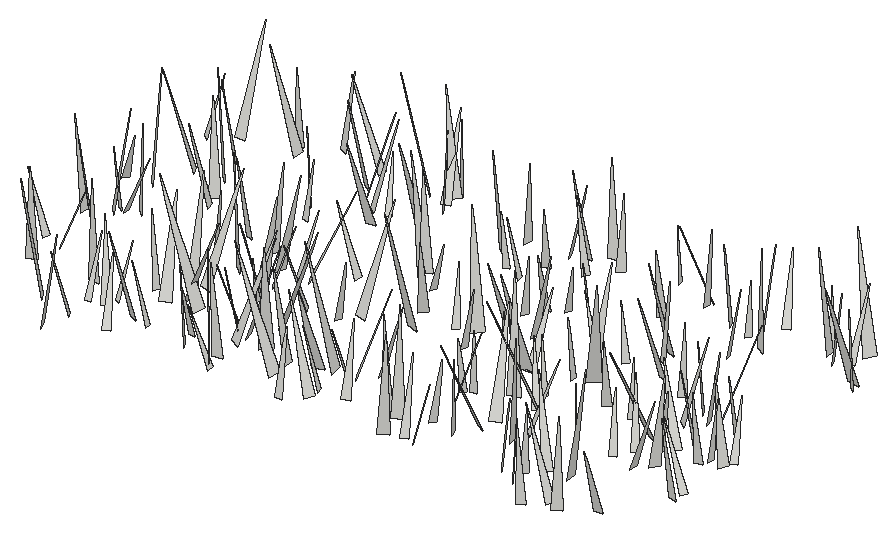
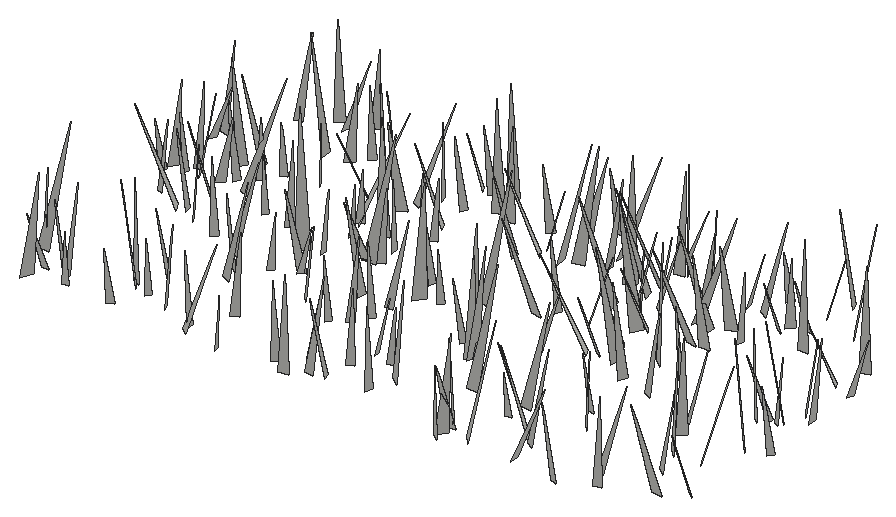
# SketchUp Ruby script. Lengths in inches.
U = 1.inch
M = Sketchup.active_model
def pt(a) = Geom::Point3d.new(a.map { |v| v * U })
def face(e, loops, mat)
  f = e.add_face(loops[0].map { |a| pt(a) })
  loops[1..].each { |l| e.add_face(l.map { |a| pt(a) }).erase! }
  f.material = f.back_material = mat if mat
  f
end
# faces: each face lists its corners as indices into pts; further lists are holes
def faces(e, pts, list, mat = nil) = list.each { |f| face(e, (f[0].is_a?(Array) ? f : [f]).map { |l| l.map { |i| pts[i] } }, mat) }
# xy, xz, yz: faces in a plane at the given z, y or x. An outline is a flat list of corners, or four numbers for a rectangle; further outlines are holes
def ring(l) = l.size == 4 ? [[l[0], l[1]], [l[2], l[1]], [l[2], l[3]], [l[0], l[3]]] : l.each_slice(2).to_a
def flat(e, list, mat, &to3) = list.each { |f| face(e, (f[0].is_a?(Array) ? f : [f]).map { |l| ring(l).map { |u, v| to3.(u, v) } }, mat) }
def xy(e, z, list, mat = nil) = flat(e, list, mat) { |x, y| [x, y, z] }
def xz(e, y, list, mat = nil) = flat(e, list, mat) { |x, z| [x, y, z] }
def yz(e, x, list, mat = nil) = flat(e, list, mat) { |y, z| [x, y, z] }
def lines(e, pts, list) = list.each { |a, b| e.add_line(pt(pts[a]), pt(pts[b])) }
# prism: a flat outline (further loops are holes) pulled along v
def prism(e, loops, v, mat = nil)
  f = face(e, loops, mat); d = Geom::Vector3d.new(v.map { |x| x * U })
  f.pushpull(f.normal.samedirection?(d) ? d.length : -d.length)
end
def box(e, o, s, mat = nil) = prism(e, [[o, [o[0] + s[0], o[1], o[2]], [o[0] + s[0], o[1] + s[1], o[2]], [o[0], o[1] + s[1], o[2]]]], [0, 0, s[2]], mat)
def at(x, y, z, deg = 0) = Geom::Transformation.translation(pt([x, y, z])) * Geom::Transformation.rotation(ORIGIN, Z_AXIS, deg.degrees)
def axes(o, x, y, z) = Geom::Transformation.new([*x, 0, *y, 0, *z, 0, *pt(o).to_a, 1])
def part(name) = M.definitions.add(name)
# library, detail: a bought-in or finely detailed component or shape, given as its bounding box
def library(name, o, s) = part(name).tap { |d| box(d.entities, o, s) }
def detail(e, o, s) = box(e.add_group.entities, o, s)
def put(e, d, t, mat = nil) = e.add_instance(d, t).tap { |i| i.material = mat if mat }
def group(e, t, mat = nil) = e.add_group.tap { |g| g.transformation = t; g.material = mat if mat }.entities
root = M.entities
c1 = part("fur_instance\#9")
p = [[0.8125,0,1.79],[0.67,-0.02,1.48],[0,-0.11,0],[0,0.11,0]]
faces(c1.entities,p,[[0,1,2,3]])
put(root,c1,axes([469.8,410.12,-21.66],[5.42096,2.25752,1.64956],[2.38588,-5.61122,-0.16143],[-1.45775,-0.7887,5.87002]))
put(root,c1,axes([536.05,411.73,-21.66],[-1.45922,4.42701,2.15741],[4.90506,1.50733,0.22462],[0.43952,-2.12407,4.65589]))
put(root,c1,axes([540.0625,413.08,-21.66],[2.8988,-5.16102,2.16058],[-5.5292,-3.01461,0.21733],[-0.85564,1.9958,5.91539]))
put(root,c1,axes([470.66,413.89,-21.66],[-3.26871,-2.2439,0.63682],[-2.29753,3.28654,-0.21245],[0.40248,0.53729,3.95909]))
put(root,c1,axes([490.34,414.11,-21.66],[-3.97846,-0.22397,0.26493],[-0.21326,3.98441,0.16592],[0.27363,-0.15114,3.9813]))
put(root,c1,axes([543.85,415.63,-21.66],[0.47232,-5.02453,0.37853],[-5.03579,-0.45765,0.20889],[0.17316,0.39615,5.04235]))
put(root,c1,axes([514.4,414.54,-21.66],[4.01557,-5.25956,2.05629],[-5.53772,-4.16187,0.169],[-1.10676,1.74125,6.61508]))
put(root,c1,axes([500.37,413.59,-21.66],[0.04059,4.23783,1.33242],[4.44047,0.00019,-0.13586],[0.12965,-1.33303,4.23585]))
put(root,c1,axes([538.44,413.93,-21.66],[-5.80532,1.01557,0.17125],[1.00882,5.80466,-0.22508],[0.20737,0.19232,5.88918]))
put(root,c1,axes([465.71,415.29,-21.66],[-6.16765,-3.82155,1.90605],[-3.98751,6.35208,-0.16723],[1.52874,1.15063,7.2537]))
put(root,c1,axes([532.24,415.05,-21.66],[-2.65775,-2.55388,1.91088],[-2.80676,3.05414,0.17806],[1.51521,1.17784,3.68161]))
put(root,c1,axes([476.0625,413.6875,-21.66],[-2.52047,3.62206,0.22803],[3.61381,2.53037,-0.24846],[0.33426,-0.04477,4.40572]))
put(root,c1,axes([489.03,415.52,-21.66],[4.97701,4.02381,2.97396],[4.34378,-5.5566,0.24873],[-2.48337,-1.65505,6.3953]))
put(root,c1,axes([518.21,415.05,-21.66],[2.97809,2.23148,0.68885],[2.24903,-3.04112,0.12836],[-0.62921,-0.30835,3.71915]))
put(root,c1,axes([489.35,416.62,-21.66],[1.40139,-5.88916,2.09043],[-6.21682,-1.53152,-0.14692],[-0.635,1.99706,6.05182]))
put(root,c1,axes([516.77,415.28,-21.66],[-2.07994,4.49979,1.08625],[4.57933,2.1742,-0.23818],[0.67657,-0.88257,4.95151]))
put(root,c1,axes([484.82,416.42,-21.66],[-3.86454,-2.68359,1.87384],[-2.96857,4.09497,-0.25773],[1.3786,1.29506,4.69786]))
put(root,c1,axes([502.83,415.91,-21.66],[-5.78073,2.46703,0.60773],[2.49572,5.79658,0.20851],[0.47643,-0.43109,6.28168]))
put(root,c1,axes([476.64,417.7,-21.66],[-2.84226,-5.05917,1.08036],[-5.16298,2.85167,-0.22901],[0.32566,1.05526,5.79838]))
put(root,c1,axes([529.49,416.57,-21.66],[3.10895,3.01642,1.49943],[3.22004,-3.26039,-0.11754],[-0.98914,-1.13301,4.33019]))
put(root,c1,axes([531.97,417.37,-21.66],[2.86459,-3.18276,1.27512],[-3.34476,-2.95943,0.1272],[-0.754,1.03614,4.28015]))
put(root,c1,axes([479.02,417.29,-21.66],[-3.86057,-0.50737,0.50019],[-0.53854,3.88252,-0.21837],[0.46646,0.28336,3.88764]))
put(root,c1,axes([496.76,417.38,-21.66],[-8.06825,0.70999,0.37952],[0.71569,8.07597,0.10667],[0.36866,-0.13964,8.09873]))
put(root,c1,axes([484.07,418.64,-21.66],[-0.05824,-3.81958,0.55077],[-3.85535,0.08183,0.15984],[0.16986,0.54776,3.81668]))
put(root,c1,axes([502.81,417.75,-21.66],[-3.79015,-1.11399,0.60809],[-1.15598,3.82064,-0.20588],[0.52388,0.37109,3.9451]))
put(root,c1,axes([513.49,418.23,-21.66],[-2.45983,6.23998,3.07468],[6.83629,2.77173,-0.15592],[1.28687,-2.79677,6.7055]))
put(root,c1,axes([506.4,417.93,-21.66],[-1.7521,4.37342,1.24469],[4.49457,1.86786,-0.23622],[0.6891,-1.06311,4.7054]))
put(root,c1,axes([511.42,418.98,-21.66],[-0.9402,5.50023,2.63792],[6.09336,0.97222,0.14463],[0.28664,-2.62629,5.57814]))
put(root,c1,axes([470.32,417.61,-21.66],[0.12612,4.07155,0.3622],[4.08216,-0.1442,0.19951],[-0.2114,-0.35539,4.06861]))
put(root,c1,axes([499.63,421.51,-21.66],[2.0561,-6.44135,0.2848],[-6.4395,-2.06652,-0.24899],[-0.32395,0.19535,6.75697]))
put(root,c1,axes([472.42,418.19,-21.66],[-4.08375,3.22336,1.0157],[3.24667,4.18417,-0.22495],[0.93853,-0.4488,5.19774]))
put(root,c1,axes([520.35,419.51,-21.66],[4.15283,1.56186,1.94961],[1.7605,-4.5132,-0.13443],[-1.7723,-0.82343,4.43479]))
put(root,c1,axes([536.68,419.74,-21.66],[7.17764,0.6661,2.04171],[0.73913,-7.45363,-0.1667],[-2.01642,-0.36113,7.20655]))
put(root,c1,axes([517.06,420,-21.66],[3.70956,-2.15387,1.10856],[-2.28011,-3.78925,0.26761],[-0.81802,0.79458,4.28116]))
put(root,c1,axes([496.37,420.23,-21.66],[-5.73495,-0.11109,1.68244],[-0.04447,5.97258,0.24275],[1.68552,-0.22038,5.73089]))
put(root,c1,axes([533.68,419.23,-21.66],[-4.18107,4.06515,1.12452],[4.17237,4.21812,0.26475],[0.61747,-0.97641,5.82552]))
put(root,c1,axes([521.83,422.34,-21.66],[-3.10911,-5.59083,0.18925],[-5.58666,3.11434,0.22319],[0.28707,0.05678,6.39328]))
put(root,c1,axes([492.43,421.375,-21.66],[4.53182,-5.76132,1.66498],[-5.89155,-4.66684,-0.11276],[-1.12014,1.237,7.32923]))
put(root,c1,axes([504.39,421.02,-21.66],[-3.02688,-2.08558,0.64094],[-2.07151,3.09116,0.27563],[0.68504,0.13224,3.66547]))
put(root,c1,axes([459.58,421.11,-21.66],[2.04038,-5.82637,1.87095],[-6.1057,-2.07021,0.21174],[-0.4092,1.83789,6.16967]))
put(root,c1,axes([472.86,419.62,-21.66],[1.48501,3.27806,0.44782],[3.28348,-1.52047,0.24164],[-0.40618,-0.30651,3.59062]))
put(root,c1,axes([468,421.49,-21.66],[0.12589,-6.48138,2.39431],[-6.90548,-0.03647,0.26437],[0.23531,2.39734,6.47721]))
put(root,c1,axes([501.4,422.42,-21.66],[-7.78363,-1.77881,1.5879],[-1.77027,7.9428,0.22014],[1.59741,0.13482,7.98126]))
put(root,c1,axes([548.46,422.96,-21.66],[-1.20745,-5.31811,1.49773],[-5.50418,1.29079,0.14593],[0.47907,1.42653,5.45151]))
put(root,c1,axes([526.46,422.29,-21.66],[-5.78196,-1.74059,3.08913],[-1.82129,6.52793,0.26926],[3.04225,0.59997,6.03227]))
put(root,c1,axes([487.04,423.0625,-21.66],[2.58883,2.26123,2.35644],[2.87323,-3.00647,-0.27159],[-1.55259,-1.79333,3.42658]))
put(root,c1,axes([488.87,420.32,-21.66],[3.08355,6.47581,0.56476],[6.50039,-3.07095,-0.27862],[0.00972,-0.62967,7.16706]))
put(root,c1,axes([489.17,422.3,-21.66],[6.39922,1.66084,0.77373],[1.68967,-6.43637,-0.15871],[-0.70856,-0.34898,6.60932]))
put(root,c1,axes([486.41,424.06,-21.66],[-2.51428,-3.3921,0.48717],[-3.39486,2.54791,0.21985],[0.4675,0.25907,4.21659]))
put(root,c1,axes([481.19,423.55,-21.66],[-8.2127,0.65784,0.53458],[0.66874,8.22786,0.14871],[0.52088,-0.19122,8.23766]))
put(root,c1,axes([504.21,422.53,-21.66],[4.71146,3.59222,0.48874],[3.58656,-4.73541,0.23065],[-0.52868,-0.11206,5.92019]))
put(root,c1,axes([478.84,424.3,-21.66],[6.32916,0.13104,0.27334],[0.13733,-6.3333,-0.14369],[-0.27023,-0.14945,6.32889]))
put(root,c1,axes([477.09,422.76,-21.66],[-2.49742,5.95651,1.04282],[6.02179,2.55284,-0.16018],[0.55273,-0.89868,6.45689]))
put(root,c1,axes([474.625,424.23,-21.66],[-4.53937,1.16522,1.40638],[1.15678,4.75002,-0.2018],[1.41333,-0.14527,4.6822]))
put(root,c1,axes([516.41,424.4,-21.66],[4.75078,2.28793,0.55209],[2.32197,-4.75936,-0.25743],[-0.38451,-0.47246,5.26671]))
put(root,c1,axes([506.1,424.72,-21.66],[4.91416,0.05831,0.74386],[0.02898,-4.96646,0.19783],[-0.74558,0.19125,4.91052]))
put(root,c1,axes([548.78,424.58,-21.66],[-4.27711,1.68369,0.0136],[1.68167,4.26988,0.26227],[-0.08344,-0.24902,4.58909]))
put(root,c1,axes([533.05,425.26,-21.66],[3.08289,1.97486,1.70839],[2.08981,-3.45082,0.21788],[-1.56569,-0.71742,3.6547]))
put(root,c1,axes([540.625,425.82,-21.66],[5.32067,-0.59583,0.38531],[-0.58759,-5.33383,-0.13414],[-0.39777,-0.09079,5.35224]))
put(root,c1,axes([487.4,425.89,-21.66],[2.96101,1.91002,1.7712],[2.18546,-3.28075,-0.11568],[-1.41742,-1.06838,3.5217]))
put(root,c1,axes([526.92,424.48,-21.66],[2.95968,3.81178,0.17357],[3.80838,-2.96454,0.16477],[-0.23661,-0.0359,4.82309]))
put(root,c1,axes([457.63,426.06,-21.66],[-4.13289,0.76106,0.51137],[0.79822,4.14817,0.27763],[0.45116,-0.36746,4.1932]))
put(root,c1,axes([460.37,425.12,-21.66],[3.48298,2.03603,0.22687],[2.02285,-3.48877,0.25421],[-0.32396,0.10555,4.02641]))
put(root,c1,axes([522.31,424.4,-21.66],[-2.78795,6.31949,0.96814],[6.36227,2.84625,-0.25738],[0.62828,-0.78026,6.90234]))
put(root,c1,axes([515.3,427.45,-21.66],[2.03457,-2.99845,1.01926],[-3.06758,-2.16697,-0.25148],[-0.78708,0.69471,3.61482]))
put(root,c1,axes([490.62,426.48,-21.66],[6.76067,1.19839,0.69108],[1.18973,-6.79585,0.14582],[-0.7059,0.02372,6.86451]))
put(root,c1,axes([542.37,427.46,-21.66],[5.43979,-3.16023,1.66658],[-3.30816,-5.60189,0.17546],[-1.34931,0.9938,6.28869]))
put(root,c1,axes([537.27,426.45,-21.66],[-1.47,3.64091,0.87512],[3.73843,1.4809,0.11844],[0.21496,-0.85654,3.92467]))
put(root,c1,axes([486.72,428.26,-21.66],[-4.48858,-3.56813,1.07524],[-3.58767,4.5928,0.2643],[1.00813,0.45789,5.72792]))
put(root,c1,axes([524.41,429.38,-21.66],[-5.605,-5.08718,0.25266],[-5.09303,5.60246,-0.18084],[0.06544,0.30374,7.56721]))
put(root,c1,axes([516.32,428,-21.66],[0.16475,-3.83195,1.51207],[-4.1166,-0.0965,0.20397],[0.15418,1.51796,3.83006]))
put(root,c1,axes([485.19,429.32,-21.66],[6.75458,-3.1446,1.55563],[-3.25939,-6.87331,0.25842],[-1.29802,0.89549,7.44621]))
put(root,c1,axes([476.94,427.67,-21.66],[-0.4945,6.57851,1.5324],[6.75453,0.47319,0.14829],[-0.03697,-1.53911,6.5954]))
put(root,c1,axes([538.65,428.65,-21.66],[-2.21571,3.96483,0.99922],[4.07213,2.24229,0.13245],[0.36886,-0.93805,4.54001]))
put(root,c1,axes([538.22,432.16,-21.66],[-2.55623,-6.61752,0.06611],[-6.61278,2.55692,0.25211],[0.25899,-0.02922,7.08959]))
put(root,c1,axes([484.28,428.47,-21.66],[3.52648,2.43175,0.31475],[2.41999,-3.54045,0.23962],[-0.3951,0.0194,4.27692]))
put(root,c1,axes([540.69,430.41,-21.66],[4.29298,-1.68508,0.76366],[-1.68331,-4.35833,-0.1541],[-0.76754,0.13347,4.60928]))
put(root,c1,axes([545.64,430.99,-21.66],[1.04102,-4.92803,1.21287],[-5.07408,-1.03535,0.14838],[-0.10125,1.21771,5.0346]))
put(root,c1,axes([524.11,429.34,-21.66],[-2.51117,3.39602,0.58609],[3.43959,2.51478,0.1658],[0.21361,-0.57041,4.22035]))
put(root,c1,axes([478.67,427.8,-21.66],[1.55056,7.17303,0.47228],[7.18686,-1.53634,-0.26142],[0.15632,-0.51668,7.33405]))
put(root,c1,axes([490.3125,431.25,-21.66],[-3.61255,-2.36918,0.54232],[-2.35627,3.65218,0.25916],[0.59592,0.07847,4.31235]))
put(root,c1,axes([520.34,430.09,-21.66],[1.64686,-6.77743,3.62945],[-7.62252,-1.92308,-0.13234],[-1.0018,3.49096,6.97339]))
put(root,c1,axes([494.48,431.53,-21.66],[4.0424,-1.6774,0.68877],[-1.67315,-4.09915,-0.16314],[-0.69903,0.11126,4.37357]))
put(root,c1,axes([544.71,431.93,-21.66],[-4.89111,-2.11302,1.38613],[-2.21595,5.03778,-0.13961],[1.21481,0.68196,5.3262]))
put(root,c1,axes([517.23,432.02,-21.66],[4.14484,0.5886,1.74948],[0.68446,-4.48393,-0.11303],[-1.71425,-0.36717,4.1849]))
put(root,c1,axes([546.34,432.375,-21.66],[4.13906,-0.88394,1.08396],[-0.87234,-4.27812,-0.15771],[-1.09332,0.06702,4.22946]))
put(root,c1,axes([548.3,432.09,-21.66],[-4.8782,2.33838,1.88669],[2.5546,5.12175,0.25721],[1.58166,-1.06025,5.40358]))
put(root,c1,axes([458.8125,432.4,-21.66],[3.31439,2.62679,2.62231],[3.03004,-3.94532,0.12232],[-2.14367,-1.5153,4.22732]))
put(root,c1,axes([523.06,432.22,-21.66],[3.01506,-0.72225,2.0256],[-1.00024,-3.559,0.21985],[-1.90373,0.72607,3.09256]))
put(root,c1,axes([541.875,431.86,-21.66],[-4.34264,3.05124,0.46122],[3.07623,4.34339,0.23041],[0.24406,-0.45414,5.3024]))
put(root,c1,axes([478.83,433.39,-21.66],[-4.49865,-5.44108,2.87885],[-5.83326,4.90701,0.15896],[1.96626,2.10876,7.05818]))
put(root,c1,axes([502.04,435.15,-21.66],[-2.39726,-7.68863,1.50052],[-7.81274,2.46126,0.12966],[0.5725,1.39306,8.05265]))
put(root,c1,axes([517.87,435.57,-21.66],[0.49777,-7.47829,0.86543],[-7.52286,-0.52678,-0.22508],[-0.28353,0.84808,7.49146]))
put(root,c1,axes([457.3,433.2,-21.66],[4.90342,0.51596,3.18153],[0.4361,-5.84514,0.27581],[-3.19346,-0.00597,4.92277]))
put(root,c1,axes([484.25,432.74,-21.66],[3.13129,2.44329,0.37399],[2.42945,-3.15346,0.26073],[-0.45532,-0.0231,3.96316]))
put(root,c1,axes([529.62,434.91,-21.66],[3.06125,-3.87557,0.82155],[-3.90702,-3.12527,-0.1848],[-0.65588,0.52812,4.93529]))
put(root,c1,axes([474.8,434.57,-21.66],[4.07501,0.67414,1.38281],[0.80205,-4.27202,-0.28088],[-1.31276,-0.5174,4.12083]))
put(root,c1,axes([548.76,433.41,-21.66],[-1.59242,3.59476,0.56652],[3.61736,1.63113,-0.18207],[0.39739,-0.44291,3.92746]))
put(root,c1,axes([533.58,434.28,-21.66],[-2.47,2.58512,1.49197],[2.74392,2.72878,-0.18549],[1.17462,-0.93843,3.57063]))
put(root,c1,axes([509.375,435.13,-21.66],[4.26328,-1.39926,0.74192],[-1.39292,-4.32659,-0.15583],[-0.75375,0.08115,4.48433]))
put(root,c1,axes([516.62,435.02,-21.66],[2.27684,-3.73592,1.683],[-3.94498,-2.51908,-0.25488],[-1.10756,1.29258,4.36763]))
put(root,c1,axes([496.08,433.37,-21.66],[1.83288,7.01444,0.75411],[7.05484,-1.82448,-0.17632],[-0.01908,-0.77421,7.24781]))
put(root,c1,axes([460.07,436.02,-21.66],[-1.89592,-3.45095,1.30694],[-3.60556,2.04518,0.16982],[0.78554,1.05823,3.9338]))
put(root,c1,axes([459.89,435.1,-21.66],[-4.21577,-3.58718,3.5566],[-4.31781,4.96325,-0.11214],[2.62178,2.40587,5.53425]))
put(root,c1,axes([482.59,436.15,-21.66],[6.6153,-1.38256,1.33275],[-1.44359,-6.733,0.18083],[-1.26639,0.45296,6.75581]))
put(root,c1,axes([525.23,438.07,-21.66],[5.72891,-5.77899,0.7373],[-5.79412,-5.75966,-0.12335],[-0.60698,0.43635,8.13646]))
put(root,c1,axes([460.98,435.99,-21.66],[4.07736,0.20577,0.16386],[0.20057,-4.0788,0.13116],[-0.17019,0.12285,4.08044]))
put(root,c1,axes([462.42,436.74,-21.66],[-3.23296,-4.09809,2.47034],[-4.47809,3.64184,0.18098],[1.68632,1.81429,5.21667]))
put(root,c1,axes([523.06,437.2,-21.66],[3.59976,0.06174,1.80471],[0.19659,-4.01441,-0.2548],[-1.79504,-0.31584,3.59126]))
put(root,c1,axes([545.87,437.55,-21.66],[-1.67476,-3.89018,1.26522],[-4.03938,1.78862,0.15259],[0.64624,1.09838,4.23261]))
put(root,c1,axes([485.2,436.09,-21.66],[2.13777,3.57515,0.4757],[3.58502,-2.16686,0.17428],[-0.39447,-0.3179,4.1619]))
put(root,c1,axes([500.69,438.7,-21.66],[3.52243,-4.25283,0.7835],[-4.27225,-3.57882,-0.21878],[-0.66956,0.46198,5.5178]))
put(root,c1,axes([518.39,435.48,-21.66],[-0.5351,4.97369,0.08314],[4.96853,0.53845,-0.2337],[0.24128,-0.05757,4.99693]))
put(root,c1,axes([486.43,436.48,-21.66],[5.74165,3.30721,0.02247],[3.30582,-5.73764,-0.2359],[0.09829,-0.21562,6.62182]))
put(root,c1,axes([538.85,436.68,-21.66],[-2.72966,-3.54913,3.67888],[-4.47058,3.67982,0.23296],[2.47878,2.72838,4.47136]))
put(root,c1,axes([505.9,437.97,-21.66],[-2.49672,2.92464,0.96124],[2.97957,2.60694,-0.1927],[0.77439,-0.6012,3.84057]))
put(root,c1,axes([540.94,438.84,-21.66],[4.61454,1.12705,1.27743],[1.23829,-4.75228,-0.2803],[-1.16993,-0.58453,4.7419]))
put(root,c1,axes([479.63,438.72,-21.66],[5.47744,-1.647,1.93505],[-1.81976,-5.75174,0.25556],[-1.77356,0.81501,5.71398]))
put(root,c1,axes([508.29,438.75,-21.66],[5.58768,-4.04107,3.86555],[-4.58295,-6.44048,-0.10822],[-3.20457,2.16447,6.89498]))
put(root,c1,axes([475.3,439.76,-21.66],[-2.10468,-4.52268,1.53831],[-4.75533,2.14388,-0.20306],[0.45584,1.48319,4.98428]))
put(root,c1,axes([539,440.18,-21.66],[-3.54566,-2.66431,1.6705],[-2.78653,3.82874,0.19209],[1.45754,0.83849,4.43096]))
put(root,c1,axes([490.47,440.07,-21.66],[-4.67838,0.58429,0.4377],[0.60816,4.68963,0.24018],[0.40387,-0.29353,4.7086]))
put(root,c1,axes([509.77,442.29,-21.66],[-0.22883,-5.12281,0.23524],[-5.12454,0.23734,0.18366],[0.19416,0.22665,5.12463]))
put(root,c1,axes([542.21,439.14,-21.66],[6.025,3.41302,0.55167],[3.40656,-6.04972,0.22351],[-0.59027,-0.07668,6.92094]))
put(root,c1,axes([456.22,441.83,-21.66],[3.1539,-2.32332,0.00557],[-2.32207,-3.15188,0.13648],[0.07647,0.11319,3.91488]))
put(root,c1,axes([534.94,441.6,-21.66],[-2.61332,3.50076,2.27341],[3.90248,3.00092,-0.13507],[1.48133,-1.72983,4.36652]))
put(root,c1,axes([513.8,442.01,-21.66],[5.74343,-0.59024,1.12729],[-0.57342,-5.85294,-0.14303],[-1.13593,-0.02976,5.77191]))
put(root,c1,axes([530.66,443.48,-21.66],[-1.81224,-5.34948,0.90018],[-5.42401,1.80193,-0.21131],[0.08596,0.92064,5.64415]))
put(root,c1,axes([467.42,442.65,-21.66],[-4.87581,-1.54153,0.97742],[-1.54685,4.96967,0.12147],[0.96896,0.17664,5.11224]))
put(root,c1,axes([498.44,443.34,-21.66],[3.31097,-1.72543,0.32906],[-1.73993,-3.31791,0.10944],[-0.24091,0.24944,3.73197]))
put(root,c1,axes([522.26,442.32,-21.66],[-3.36159,2.04077,0.19725],[2.04893,3.35754,0.1809],[0.07444,-0.25709,3.9284]))
put(root,c1,axes([459.37,442.58,-21.66],[4.78863,4.89843,2.46119],[5.13986,-5.14824,0.24599],[-1.90629,-1.57608,6.84581]))
put(root,c1,axes([522.34,441.88,-21.66],[-0.07417,5.83715,1.21265],[5.95855,0.11247,-0.17697],[0.19614,-1.2097,5.83493]))
put(root,c1,axes([525.3125,443.69,-21.66],[-2.21806,2.84038,1.31516],[3.07662,2.27502,0.2754],[0.57601,-1.21396,3.59328]))
put(root,c1,axes([509.79,445.23,-21.66],[3.72524,-2.31212,0.81738],[-2.32656,-3.80205,-0.15146],[-0.77532,0.29988,4.38182]))
put(root,c1,axes([466.73,444.4375,-21.66],[3.45962,-4.50001,2.91683],[-5.02174,-3.93643,-0.1168],[-1.88153,2.2319,5.67498]))
put(root,c1,axes([495.38,445.46,-21.66],[-7.11208,1.53537,2.26223],[1.65379,7.4363,0.15223],[2.17716,-0.6331,7.27433]))
put(root,c1,axes([495.52,445.7,-21.66],[3.10657,-5.20372,2.6425],[-5.63717,-3.45056,-0.16782],[-1.51121,2.17421,6.05816]))
put(root,c1,axes([511.11,447.47,-21.66],[1.53045,-4.60076,0.23907],[-4.60681,-1.52625,0.11946],[0.03806,0.26453,4.84716]))
put(root,c1,axes([518.17,446.57,-21.66],[-3.06281,-3.15709,1.43812],[-3.29391,3.24851,0.11628],[1.08883,0.94666,4.3971]))
put(root,c1,axes([528.46,446.27,-21.66],[-2.24155,-3.80564,2.54295],[-4.42537,2.52493,-0.12217],[1.16862,2.26183,4.41503]))
put(root,c1,axes([461.24,447.79,-21.66],[-5.49942,-3.45806,0.94275],[-3.51329,5.5426,-0.16378],[0.70973,0.64178,6.49422]))
put(root,c1,axes([477.7,446.68,-21.66],[1.06055,3.50039,1.15885],[3.68372,-1.05849,-0.17402],[-0.16095,-1.16074,3.65339]))
put(root,c1,axes([527.93,448.32,-21.66],[-2.71876,-5.31687,1.33657],[-5.469,2.73415,-0.24823],[0.3815,1.3048,5.9665]))
put(root,c1,axes([464.92,448.27,-21.66],[4.55418,4.59674,3.34406],[5.23121,-5.06575,-0.16086],[-2.22422,-2.50228,6.46875]))
put(root,c1,axes([513.14,448.69,-21.66],[3.09975,-1.98369,0.33098],[-1.98147,-3.11644,-0.1208],[-0.34401,0.07615,3.67817]))
put(root,c1,axes([483.9,450.47,-21.66],[0.0355,-6.28923,0.69696],[-6.32457,-0.05728,-0.19472],[-0.19984,0.69551,6.28631]))
put(root,c1,axes([491.09,450.92,-21.66],[-1.0754,-7.3325,1.08617],[-7.40599,1.10888,0.15329],[0.31086,1.05196,7.40935]))
put(root,c1,axes([475.96,449.7,-21.66],[3.3067,2.95122,2.18217],[3.23124,-3.73382,0.15332],[-1.74087,-1.32466,4.4295]))
put(root,c1,axes([504.39,451.2,-21.66],[-3.7389,-0.44853,0.79303],[-0.43438,3.82202,0.11371],[0.80087,-0.02096,3.764]))
put(root,c1,axes([463.32,452.23,-21.66],[-2.97615,-4.05495,1.48787],[-4.26463,3.04523,-0.23114],[0.68511,1.34083,5.02461]))
put(root,c1,axes([501.67,452.18,-21.66],[0.6335,-3.36408,1.34348],[-3.58683,-0.77327,-0.24494],[-0.50657,1.2682,3.41444]))
put(root,c1,axes([533.28,451.81,-21.66],[4.00682,1.30969,1.18737],[1.29487,-4.17692,0.23764],[-1.20352,-0.13365,4.20874]))
put(root,c1,axes([547.74,455.72,-21.66],[-0.40558,-7.48594,0.6627],[-7.51279,0.42075,0.15485],[0.19107,0.65318,7.49532]))
put(root,c1,axes([521.9,454.26,-21.66],[2.34766,-4.1804,1.05082],[-4.25289,-2.44131,-0.21062],[-0.70205,0.80976,4.78987]))
put(root,c1,axes([505.07,454.9375,-21.66],[1.42662,-4.11071,0.89066],[-4.20545,-1.41051,0.22612],[-0.07357,0.91596,4.34535]))
put(root,c1,axes([484.17,453.18,-21.66],[-1.12302,3.48075,0.37457],[3.50037,1.10997,0.18007],[-0.0574,-0.41163,3.65299]))
put(root,c1,axes([498.94,454.73,-21.66],[3.12486,4.78234,3.10342],[5.39282,-3.6275,0.15986],[-1.8492,-2.49745,5.71052]))
put(root,c1,axes([482,453.15,-21.66],[3.27247,4.57721,0.86039],[4.6176,-3.3258,0.13012],[-0.60735,-0.62316,5.62521]))
put(root,c1,axes([548.35,454.65,-21.66],[-3.07714,-3.38347,1.94932],[-3.73457,3.27489,-0.21099],[1.14047,1.59489,4.5686]))
put(root,c1,axes([535.08,455.16,-21.66],[-2.81459,-5.30869,2.75415],[-5.79641,3.17103,0.18862],[1.47279,2.33491,6.00571]))
put(root,c1,axes([457.4375,454.41,-21.66],[2.29816,3.3477,0.63042],[3.39972,-2.30202,-0.16916],[-0.21536,-0.61617,4.05709]))
put(root,c1,axes([478.39,456.68,-21.66],[-3.05463,-4.97038,1.37571],[-5.09206,3.16016,0.11108],[0.81742,1.11209,5.83293]))
put(root,c1,axes([479.4375,455.46,-21.66],[5.1332,2.66859,0.80867],[2.72409,-5.16107,-0.26035],[-0.59552,-0.60587,5.77956]))
put(root,c1,axes([534.64,455.86,-21.66],[5.13574,3.88277,2.0176],[4.11622,-5.34233,-0.19668],[-1.48436,-1.3806,6.4353]))
put(root,c1,axes([532.21,456.64,-21.66],[-2.65217,1.9255,1.58872],[2.09556,2.97695,-0.10973],[1.35655,-0.83418,3.2756]))
put(root,c1,axes([509.6,456.23,-21.66],[-4.39525,1.44739,0.73649],[1.42922,4.45652,-0.22883],[0.77116,-0.01,4.62177]))
put(root,c1,axes([529.07,457.5,-21.66],[4.09073,2.15745,2.5023],[2.51133,-4.61824,-0.12369],[-2.14694,-1.2913,4.62314]))
put(root,c1,axes([467.84,457.75,-21.66],[-6.68615,-0.01766,0.93467],[0.01232,6.74773,0.2156],[0.93476,-0.21523,6.6827]))
put(root,c1,axes([488.25,457.8,-21.66],[-3.74017,-2.83655,2.38458],[-3.12746,4.23356,0.13062],[1.98777,1.32365,4.69232]))
put(root,c1,axes([499.97,458.0625,-21.66],[-4.58199,0.67037,2.42399],[0.81188,5.16228,0.10702],[2.38033,-0.47034,4.62953]))
put(root,c1,axes([543.2,457.83,-21.66],[3.76786,2.01641,1.4087],[2.07515,-3.9894,0.15999],[-1.32064,-0.51569,4.27049]))
put(root,c1,axes([507.41,459.375,-21.66],[-0.73911,-5.79285,1.55471],[-5.99778,0.70592,-0.22109],[-0.03032,1.57006,5.83563]))
put(root,c1,axes([466.78,459.3,-21.66],[0.54293,-5.17192,1.62827],[-5.42158,-0.49338,0.24063],[0.08095,1.64396,5.19477]))
put(root,c1,axes([460.59,456.47,-21.66],[0.90222,6.95991,0.72818],[6.98982,-0.93156,0.24337],[-0.33621,-0.69025,7.01392]))
put(root,c1,axes([524.17,460.4,-21.66],[-3.22391,-4.50813,0.36238],[-4.51102,3.23719,0.13952],[0.32445,0.21334,5.54053]))
put(root,c1,axes([505.49,458.62,-21.66],[4.51759,1.55237,1.02195],[1.60919,-4.61101,-0.10928],[-0.92991,-0.4377,4.77562]))
put(root,c1,axes([484.55,459.95,-21.66],[-5.73221,-5.07274,1.73381],[-5.23258,5.8463,-0.19467],[1.1657,1.29813,7.652]))
put(root,c1,axes([541.58,459.26,-21.66],[-6.14594,-1.15799,1.95321],[-1.28361,6.42082,-0.2323],[1.87305,0.60056,6.24977]))
put(root,c1,axes([512.07,459.37,-21.66],[-2.98009,3.50221,2.17702],[3.82104,3.35523,-0.16707],[1.55067,-1.53712,4.59549]))
put(root,c1,axes([524.23,459.25,-21.66],[4.53301,0.32886,1.81446],[0.26511,-4.88148,0.22244],[-1.82486,0.10775,4.53948]))
put(root,c1,axes([477.6875,460.22,-21.66],[-5.92651,0.06077,0.05927],[0.05827,5.92175,-0.24529],[0.06173,0.24468,5.92174]))
put(root,c1,axes([544.89,458.88,-21.66],[0.14678,4.73777,0.12743],[4.7339,-0.15274,0.22615],[-0.23006,-0.12022,4.73465]))
put(root,c1,axes([540.88,460.39,-21.66],[-1.02276,3.4571,1.0392],[3.60758,1.01767,0.16502],[0.12981,-1.04418,3.60144]))
put(root,c1,axes([509.66,461.02,-21.66],[-1.05184,5.80364,2.59591],[6.34975,1.09094,0.13387],[0.3189,-2.57972,5.89666]))
put(root,c1,axes([487.54,460.73,-21.66],[-5.4066,3.91291,1.98693],[4.14231,5.59139,0.26032],[1.44915,-1.38406,6.66892]))
put(root,c1,axes([487.61,459.06,-21.66],[-1.13883,5.42731,0.08742],[5.42427,1.13458,0.2244],[-0.2017,-0.13157,5.54096]))
put(root,c1,axes([518.83,461.39,-21.66],[3.01328,1.01562,1.71575],[1.06477,-3.44849,0.1713],[-1.68569,-0.36275,3.17522]))
put(root,c1,axes([471.23,461.46,-21.66],[1.95636,4.4496,1.57567],[4.70552,-1.97342,-0.26957],[-0.3738,-1.55425,4.8532]))
put(root,c1,axes([487.67,461.73,-21.66],[2.36348,3.65871,1.87372],[3.9267,-2.64879,0.21906],[-1.21573,-1.4425,4.3502]))
put(root,c1,axes([534.37,460.61,-21.66],[-2.34195,3.99616,0.3444],[3.99913,2.35703,-0.15486],[0.30802,-0.21845,4.62925]))
put(root,c1,axes([545.4,461.52,-21.66],[-6.9298,2.98954,1.57704],[3.02348,7.09089,-0.15622],[1.51094,-0.47802,7.54553]))
